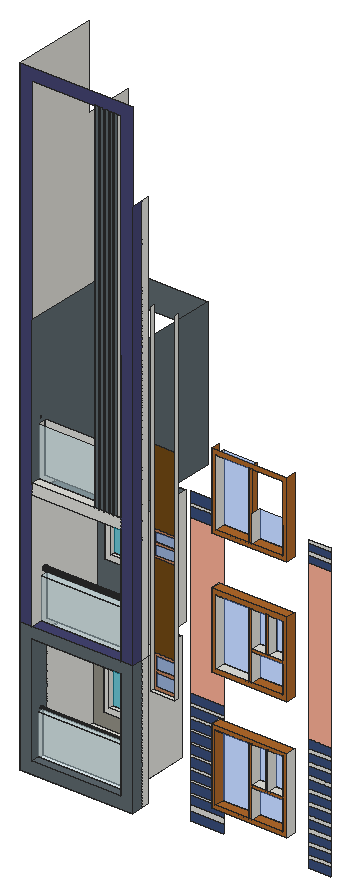
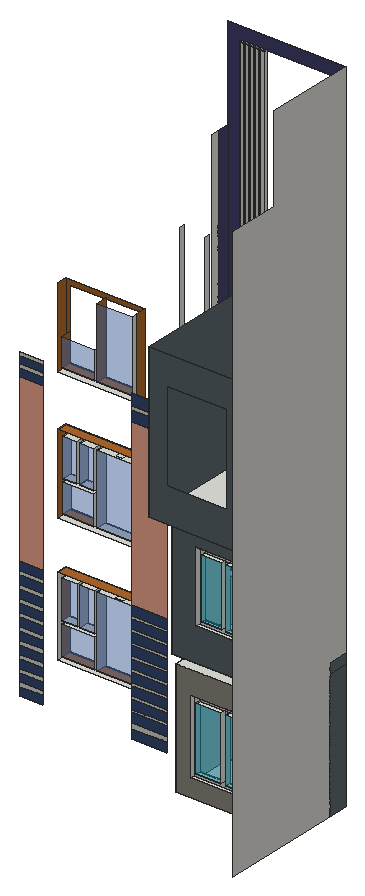
# SketchUp Ruby script. Lengths in inches.
U = 1.inch
M = Sketchup.active_model
def pt(a) = Geom::Point3d.new(a.map { |v| v * U })
def face(e, loops, mat)
  f = e.add_face(loops[0].map { |a| pt(a) })
  loops[1..].each { |l| e.add_face(l.map { |a| pt(a) }).erase! }
  f.material = f.back_material = mat if mat
  f
end
# faces: each face lists its corners as indices into pts; further lists are holes
def faces(e, pts, list, mat = nil) = list.each { |f| face(e, (f[0].is_a?(Array) ? f : [f]).map { |l| l.map { |i| pts[i] } }, mat) }
# xy, xz, yz: faces in a plane at the given z, y or x. An outline is a flat list of corners, or four numbers for a rectangle; further outlines are holes
def ring(l) = l.size == 4 ? [[l[0], l[1]], [l[2], l[1]], [l[2], l[3]], [l[0], l[3]]] : l.each_slice(2).to_a
def flat(e, list, mat, &to3) = list.each { |f| face(e, (f[0].is_a?(Array) ? f : [f]).map { |l| ring(l).map { |u, v| to3.(u, v) } }, mat) }
def xy(e, z, list, mat = nil) = flat(e, list, mat) { |x, y| [x, y, z] }
def xz(e, y, list, mat = nil) = flat(e, list, mat) { |x, z| [x, y, z] }
def yz(e, x, list, mat = nil) = flat(e, list, mat) { |y, z| [x, y, z] }
def lines(e, pts, list) = list.each { |a, b| e.add_line(pt(pts[a]), pt(pts[b])) }
# prism: a flat outline (further loops are holes) pulled along v
def prism(e, loops, v, mat = nil)
  f = face(e, loops, mat); d = Geom::Vector3d.new(v.map { |x| x * U })
  f.pushpull(f.normal.samedirection?(d) ? d.length : -d.length)
end
def box(e, o, s, mat = nil) = prism(e, [[o, [o[0] + s[0], o[1], o[2]], [o[0] + s[0], o[1] + s[1], o[2]], [o[0], o[1] + s[1], o[2]]]], [0, 0, s[2]], mat)
def at(x, y, z, deg = 0) = Geom::Transformation.translation(pt([x, y, z])) * Geom::Transformation.rotation(ORIGIN, Z_AXIS, deg.degrees)
def axes(o, x, y, z) = Geom::Transformation.new([*x, 0, *y, 0, *z, 0, *pt(o).to_a, 1])
def part(name) = M.definitions.add(name)
# library, detail: a bought-in or finely detailed component or shape, given as its bounding box
def library(name, o, s) = part(name).tap { |d| box(d.entities, o, s) }
def detail(e, o, s) = box(e.add_group.entities, o, s)
def put(e, d, t, mat = nil) = e.add_instance(d, t).tap { |i| i.material = mat if mat }
def group(e, t, mat = nil) = e.add_group.tap { |g| g.transformation = t; g.material = mat if mat }.entities
root = M.entities
M.materials.add("[Blinds Weave]").color = [114, 74, 20]
M.materials.add("[Color B02]").color = [255, 178, 153]
M.materials.add("[Color I02]").color = [68, 68, 114]
M.materials.add("[Formica Blue]").color = [58, 79, 124]
M.materials.add("[Formica Graystone]").color = [149, 146, 135]
M.materials.add("[Formica Speckled Grey]").color = [94, 105, 111]
M.materials.add("[Terrazzo Tile Light]").color = [219, 217, 210]
M.materials.add("[Translucent Glass Blue]").color = [100, 149, 237]
M.materials["[Translucent Glass Blue]"].alpha = 0.5
M.materials.add("[Translucent Glass Safety]").color = [204, 235, 244]
M.materials["[Translucent Glass Safety]"].alpha = 0.5
M.materials.add("[Translucent Glass Tinted]").color = [8, 201, 241]
M.materials["[Translucent Glass Tinted]"].alpha = 0.48
M.materials.add("[Wood Bamboo]").color = [177, 105, 43]
M.materials.add("[Wood Veneer 02]").color = [190, 128, 91]
xy(root,279.75,[[0,7.5,0,18.26,13.78,18.26,13.78,61.625,320.63,61.625,320.63,7.5]])
xy(root,313.07,[[33.32,45.54,287.32,227.125]])
xy(root,313.07,[[33.32,7.5,287.32,29.45]],"[Formica Speckled Grey]")
xy(root,360.6875,[[72.83,214.5625,246.76,227.125]])
xy(root,376.26,[[88.4,214.5625,150.48,227.125],[164.58,214.5625,231.1875,227.125]])
xy(root,378.36,[[552.31,0,767.87,28.0625]])
xy(root,389.26,[[563.2,0,660.09,28.0625],[667.35,0,756.97,28.0625]],"[Wood Bamboo]")
xy(root,429.69,[[33.32,29.45,287.32,45.54]],"[Translucent Glass Safety]")
xy(root,470.05,[[667.35,0,756.97,28.0625]])
xy(root,477.65,[[667.35,0,708.74,28.0625],[713.89,0,756.97,28.0625]])
xy(root,548.74,[[88.4,214.5625,150.48,227.125],[164.58,214.5625,231.1875,227.125]])
xy(root,564.3125,[[72.83,214.5625,246.76,227.125]])
xy(root,583.02,[[[563.2,0,660.09,28.0625],[593.19,6.08,612.69,23.46]],[667.35,0,708.74,28.0625],[713.89,0,756.97,28.0625],[593.19,6.08,612.69,23.46]])
xy(root,586.3125,[[345.55,40.625,414.87,53.5625]])
xy(root,593.92,[[552.31,0,767.87,28.0625]],"[Wood Bamboo]")
xy(root,626.26,[[0,7.5,33.32,61.625],[[33.32,7.5,287.32,61.625],[52.66,20.59,85.91,47.84],[228.16,20.59,261.41,47.84]],[52.66,20.59,85.91,47.84],[228.16,20.59,261.41,47.84],[33.32,61.625,287.32,227.125]])
xy(root,656.21,[[33.32,61.625,287.32,239.5625]])
xy(root,656.21,[[33.32,7.5,287.32,41.42]],"[Color I02]")
xy(root,726.11,[[552.31,0,767.87,28.0625]])
xy(root,738.9,[[565.1,0,660.09,28.0625]])
xy(root,738.9,[[669.04,0,755.07,28.0625]],"[Wood Bamboo]")
xy(root,745.45,[[66.75,227.8125,221.75,239.5625]])
xy(root,760.3,[[81.6,227.8125,139.43,239.5625],[152.36,227.8125,206.9,239.5625]])
xy(root,772.03,[[33.32,41.42,287.32,61.625]],"[Translucent Glass Safety]")
xy(root,817.79,[[669.04,0,755.07,28.0625]])
xy(root,825.96,[[669.04,0,707.54,28.0625],[715.14,0,755.07,28.0625]])
xy(root,925.04,[[81.6,227.8125,139.43,239.5625],[152.36,227.8125,206.9,239.5625]])
xy(root,928.88,[[[565.1,0,660.09,28.0625],[593.45,6.63,615.57,23.07]],[669.04,0,707.54,28.0625],[715.14,0,755.07,28.0625],[593.45,6.63,615.57,23.07]])
xy(root,939.89,[[66.75,227.8125,221.75,239.5625]])
xy(root,941.67,[[552.31,0,767.87,28.0625]],"[Wood Bamboo]")
xy(root,993.38,[[53.13,32.7,79.76,59.32],[228.95,32.7,255.57,59.32],[49.26,183.32,75.88,209.95],[228.95,183.32,255.57,209.95]])
xy(root,993.38,[[[33.32,7.5,287.32,239.5625],[53.13,32.7,79.76,59.32],[228.95,32.7,255.57,59.32],[228.95,183.32,255.57,209.95],[49.26,183.32,75.88,209.95]]],"[Formica Speckled Grey]")
xy(root,1023.34,[[33.32,7.5,213.36,7.5,213.36,17.375,224.6,17.375,224.6,7.5,227.11,7.5,227.11,17.375,238.35,17.375,238.35,7.5,241.05,7.5,241.05,17.375,252.29,17.375,252.29,7.5,255.11,7.5,255.11,17.375,266.35,17.375,266.35,7.5,269.11,7.5,269.11,17.375,280.35,17.375,280.35,7.5,287.32,7.5,287.32,31.52,33.32,31.52],[213.36,7.5,224.6,17.375],[227.11,7.5,238.35,17.375],[241.05,7.5,252.29,17.375],[255.11,7.5,266.35,17.375],
  [269.11,7.5,280.35,17.375],[33.32,55.75,287.32,318.5]])
xy(root,1082.8,[[552.31,0,767.87,28.0625]])
xy(root,1094.55,[[564.0625,0,660.09,28.0625],[667.45,0,756.11,28.0625]],"[Wood Bamboo]")
xz(root,0,[[[552.31,378.36,767.87,593.92],[563.2,389.26,756.97,583.02]],[660.09,389.26,667.35,583.02],[667.35,470.05,756.97,477.65],[708.74,477.65,713.89,583.02],[[552.31,726.11,767.87,941.67],[565.1,738.9,755.07,928.88]],
  [660.09,738.9,669.04,928.88],[669.04,817.79,755.07,825.96],[707.54,825.96,715.14,928.88],[[552.31,1082.8,767.87,1298.36],[564.0625,1094.55,756.11,1286.6]],[660.09,1094.55,667.45,1286.6]],"[Wood Bamboo]")
xz(root,7.5,[[33.32,993.38,287.32,1023.34]])
xz(root,7.5,[[0,656.21,33.32,656.21,33.32,2052.75,287.32,2052.75,287.32,656.21,320.63,656.21,320.63,2087.5625,0,2087.5625]],"[Color I02]")
xz(root,7.5,[[0,279.75,320.63,279.75,320.63,656.21,0,656.21,0,626.26,287.32,626.26,287.32,313.07,33.32,313.07,33.32,626.26,0,626.26],[213.36,1023.34,224.6,2052.75],[227.11,1023.34,238.35,2052.75],[241.05,1023.34,252.29,2052.75],[255.11,1023.34,266.35,2052.75],
  [269.11,1023.34,280.35,2052.75]],"[Formica Speckled Grey]")
xz(root,17.375,[[213.36,1023.34,224.6,2052.75],[227.11,1023.34,238.35,2052.75],[241.05,1023.34,252.29,2052.75],[255.11,1023.34,266.35,2052.75],[269.11,1023.34,280.35,2052.75]])
xz(root,28.0625,[[563.2,389.26,660.09,583.02],[667.35,389.26,756.97,470.05],[667.35,477.65,708.74,583.02],[713.89,477.65,756.97,583.02],[565.1,738.9,660.09,928.88],
  [669.04,738.9,755.07,817.79],[669.04,825.96,707.54,928.88],[715.14,825.96,755.07,928.88],[564.0625,1094.55,660.09,1286.6],[667.45,1094.55,756.11,1171.56]],"[Translucent Glass Blue]")
xz(root,29.45,[[33.32,313.07,287.32,429.69]],"[Translucent Glass Safety]")
xz(root,31.52,[[33.32,1023.34,287.32,1165.4]],"[Translucent Glass Safety]")
xz(root,41.42,[[33.32,656.21,287.32,772.03]],"[Translucent Glass Safety]")
xz(root,45.54,[[33.32,313.07,287.32,429.69]])
xz(root,53.5625,[[345.55,680.48,414.87,923.58],[345.55,998.27,414.87,1212.67]],"[Blinds Weave]")
xz(root,53.5625,[[353.15,593.91,407.27,630.07],[353.15,639.46,407.27,672.89],[352.13,930.16,408.29,958.03],[352.13,964.22,408.29,991.69]],"[Translucent Glass Blue]")
xz(root,53.5625,[[[345.55,586.3125,414.87,680.48],[353.15,593.91,407.27,672.89]],[353.15,630.07,407.27,639.46],[[345.55,923.58,414.87,998.27],[352.13,930.16,408.29,991.69]],[352.13,958.03,408.29,964.22]],"[Wood Veneer 02]")
xz(root,55.75,[[33.32,1023.34,287.32,1165.4]])
xz(root,61.625,[[782.27,302.4,843.32,312.28],[443.82,306.77,538.37,320.57],[782.27,335.77,843.32,346.28],[443.82,346.58,538.37,353.19],[782.27,369.77,843.32,380.28],
  [443.82,379.21,538.37,385.82],[782.27,403.77,843.32,414.28],[443.82,411.83,538.37,418.44],[782.27,437.77,843.32,448.28],[443.82,444.46,538.37,451.07],
  [782.27,471.77,843.32,482.28],[443.82,477.08,538.37,483.69],[782.27,505.77,843.32,516.28],[443.82,509.71,538.37,516.32],[782.27,539.77,843.32,550.28],
  [443.82,542.33,538.37,548.94],[782.27,573.77,843.32,584.28],[443.82,574.96,538.37,581.57],[33.32,656.21,287.32,772.03],[782.27,1079.01,843.32,1088.41],
  [443.82,1085.07,538.37,1094.19],[782.27,1109.47,843.32,1118.875]])
xz(root,61.625,[[443.82,607.58,538.37,1053.88],[782.27,607.77,843.32,1057.95]],"[Color B02]")
xz(root,61.625,[[782.27,278.91,843.32,302.4],[443.82,280.75,538.37,306.77],[782.27,312.28,843.32,335.77],[443.82,320.57,538.37,346.58],[782.27,346.28,843.32,369.77],
  [443.82,353.19,538.37,379.21],[782.27,380.28,843.32,403.77],[443.82,385.82,538.37,411.83],[782.27,414.28,843.32,437.77],[443.82,418.44,538.37,444.46],
  [782.27,448.28,843.32,471.77],[443.82,451.07,538.37,477.08],[782.27,482.28,843.32,505.77],[443.82,483.69,538.37,509.71],[782.27,516.28,843.32,539.77],
  [443.82,516.32,538.37,542.33],[443.82,548.94,538.37,574.96],[782.27,550.28,843.32,573.77],[443.82,581.57,538.37,607.58],[782.27,584.28,843.32,607.77],
  [443.82,1053.88,538.37,1085.07],[782.27,1057.95,843.32,1079.01],[782.27,1088.41,843.32,1109.47],[443.82,1094.19,538.37,1125.38]],"[Formica Blue]")
xz(root,214.5625,[[[72.83,360.6875,246.76,564.3125],[88.4,376.26,231.1875,548.74]],[150.48,376.26,164.58,548.74]])
xz(root,227.125,[[[33.32,313.07,287.32,626.26],[72.83,360.6875,246.76,564.3125]]],"[Formica Graystone]")
xz(root,227.125,[[88.4,376.26,150.48,548.74],[164.58,376.26,231.1875,548.74]],"[Translucent Glass Tinted]")
xz(root,227.8125,[[[66.75,745.45,221.75,939.89],[81.6,760.3,206.9,925.04]],[139.43,760.3,152.36,925.04]])
xz(root,239.5625,[[[33.32,656.21,287.32,993.38],[66.75,745.45,221.75,939.89]]],"[Formica Speckled Grey]")
xz(root,239.5625,[[81.6,760.3,139.43,925.04],[152.36,760.3,206.9,925.04]],"[Translucent Glass Tinted]")
xz(root,318.5,[[[33.32,1023.34,287.32,1439.76],[74.41,1117.04,237.41,1361.98]]],"[Formica Speckled Grey]")
yz(root,0,[[7.5,279.75,61.625,626.26],[7.5,626.26,61.625,656.21]],"[Formica Speckled Grey]")
yz(root,0,[[61.625,279.75,61.625,656.21,7.5,656.21,7.5,2087.5625,252.1,2087.5625,252.1,1852.125,391.54,1852.125,391.54,279.75]],"[Terrazzo Tile Light]")
yz(root,33.32,[[61.625,313.07,227.125,626.26],[[7.5,656.21,41.42,656.21,41.42,772.03,61.625,772.03,61.625,656.21,239.5625,656.21,239.5625,993.38,7.5,993.38],[50.17,783.1,48.47,783.32,46.89,783.98,45.53,785.02,44.49,786.38,43.83,787.97,43.61,789.66,43.83,791.36,44.49,792.94,45.53,794.3,46.89,795.35,48.47,796,50.17,796.23,51.87,796,53.45,795.35,54.8125,794.3,55.86,792.94,56.51,791.36,56.74,789.66,56.51,787.97,55.86,786.38,54.8125,785.02,53.45,783.98,51.87,783.32]]])
yz(root,33.32,[[[7.5,313.07,29.45,313.07,29.45,429.69,45.54,429.69,45.54,313.07,61.625,313.07,61.625,626.26,7.5,626.26],[37.49,435.16,36.68,435.27,35.93,435.58,35.28,436.08,34.78,436.72,34.47,437.48,34.37,438.28,34.47,439.09,34.78,439.85,35.28,440.49,35.93,440.99,36.68,441.3,37.49,441.41,38.3,441.3,39.05,440.99,39.7,440.49,40.2,439.85,40.51,439.09,40.62,438.28,40.51,437.48,40.2,436.72,39.7,436.08,39.05,435.58,38.3,435.27]],[[7.5,1023.34,31.52,1023.34,31.52,1165.4,55.75,1165.4,55.75,1023.34,318.5,1023.34,318.5,1439.76,7.5,1439.76],[40.12,1173.19,38.74,1173.37,37.46,1173.9,36.36,1174.75,35.52,1175.85,34.99,1177.13,34.81,1178.5,34.99,1179.88,35.52,1181.16,36.36,1182.26,37.46,1183.1,38.74,1183.63,40.12,1183.82,41.49,1183.63,42.77,1183.1,43.875,1182.26,44.72,1181.16,45.25,1179.88,45.43,1178.5,45.25,1177.13,44.72,1175.85,43.875,1174.75,42.77,1173.9,41.49,1173.37]]],"[Formica Speckled Grey]")
yz(root,66.75,[[227.8125,745.45,239.5625,939.89]])
yz(root,72.83,[[214.5625,360.6875,227.125,564.3125]])
yz(root,81.6,[[227.8125,760.3,239.5625,925.04]])
yz(root,88.4,[[214.5625,376.26,227.125,548.74]])
yz(root,139.43,[[227.8125,760.3,239.5625,925.04]])
yz(root,150.48,[[214.5625,376.26,227.125,548.74]])
yz(root,152.36,[[227.8125,760.3,239.5625,925.04]])
yz(root,164.58,[[214.5625,376.26,227.125,548.74]])
yz(root,206.9,[[227.8125,760.3,239.5625,925.04]])
yz(root,213.36,[[7.5,1023.34,17.375,2052.75]])
yz(root,221.75,[[227.8125,745.45,239.5625,939.89]])
yz(root,224.6,[[7.5,1023.34,17.375,2052.75]])
yz(root,227.11,[[7.5,1023.34,17.375,2052.75]])
yz(root,231.1875,[[214.5625,376.26,227.125,548.74]])
yz(root,238.35,[[7.5,1023.34,17.375,2052.75]])
yz(root,241.05,[[7.5,1023.34,17.375,2052.75]])
yz(root,246.76,[[214.5625,360.6875,227.125,564.3125]])
yz(root,252.29,[[7.5,1023.34,17.375,2052.75]])
yz(root,255.11,[[7.5,1023.34,17.375,2052.75]])
yz(root,266.35,[[7.5,1023.34,17.375,2052.75]])
yz(root,269.11,[[7.5,1023.34,17.375,2052.75]])
yz(root,280.35,[[7.5,1023.34,17.375,2052.75]])
yz(root,287.32,[[61.625,313.07,227.125,626.26],[37.49,435.16,38.3,435.27,39.05,435.58,39.7,436.08,40.2,436.72,40.51,437.48,40.62,438.28,40.51,439.09,40.2,439.85,39.7,440.49,39.05,440.99,38.3,441.3,37.49,441.41,36.68,441.3,35.93,440.99,35.28,440.49,34.78,439.85,34.47,439.09,34.37,438.28,34.47,437.48,34.78,436.72,35.28,436.08,35.93,435.58,36.68,435.27],[[7.5,656.21,7.5,993.38,239.5625,993.38,239.5625,656.21,61.625,656.21,61.625,772.03,41.42,772.03,41.42,656.21],[50.17,783.1,51.87,783.32,53.45,783.98,54.8125,785.02,55.86,786.38,56.51,787.97,56.74,789.66,56.51,791.36,55.86,792.94,54.8125,794.3,53.45,795.35,51.87,796,50.17,796.23,48.47,796,46.89,795.35,45.53,794.3,44.49,792.94,43.83,791.36,43.61,789.66,43.83,787.97,44.49,786.38,45.53,785.02,46.89,783.98,48.47,783.32]],[50.17,783.1,51.87,783.32,53.45,783.98,54.8125,785.02,55.86,786.38,56.51,787.97,56.74,789.66,56.51,791.36,55.86,792.94,54.8125,794.3,53.45,795.35,51.87,796,50.17,796.23,48.47,796,46.89,795.35,45.53,794.3,44.49,792.94,43.83,791.36,43.61,789.66,43.83,787.97,44.49,786.38,45.53,785.02,46.89,783.98,48.47,783.32]])
yz(root,287.32,[[[7.5,313.07,7.5,626.26,61.625,626.26,61.625,313.07,45.54,313.07,45.54,429.69,29.45,429.69,29.45,313.07],[37.49,435.16,38.3,435.27,39.05,435.58,39.7,436.08,40.2,436.72,40.51,437.48,40.62,438.28,40.51,439.09,40.2,439.85,39.7,440.49,39.05,440.99,38.3,441.3,37.49,441.41,36.68,441.3,35.93,440.99,35.28,440.49,34.78,439.85,34.47,439.09,34.37,438.28,34.47,437.48,34.78,436.72,35.28,436.08,35.93,435.58,36.68,435.27]],[[7.5,1023.34,7.5,1439.76,318.5,1439.76,318.5,1023.34,55.75,1023.34,55.75,1165.4,31.52,1165.4,31.52,1023.34],[40.12,1173.19,41.49,1173.37,42.77,1173.9,43.875,1174.75,44.72,1175.85,45.25,1177.13,45.43,1178.5,45.25,1179.88,44.72,1181.16,43.875,1182.26,42.77,1183.1,41.49,1183.63,40.12,1183.82,38.74,1183.63,37.46,1183.1,36.36,1182.26,35.52,1181.16,34.99,1179.88,34.81,1178.5,34.99,1177.13,35.52,1175.85,36.36,1174.75,37.46,1173.9,38.74,1173.37]]],"[Formica Speckled Grey]")
yz(root,320.63,[[40.625,279.75,61.625,656.21],[40.625,656.21,61.625,1831.875]])
yz(root,320.63,[[7.5,656.21,40.625,1831.875]],"[Color I02]")
yz(root,320.63,[[7.5,279.75,40.625,656.21]],"[Formica Speckled Grey]")
yz(root,345.55,[[40.625,586.3125,53.5625,1568.875]])
yz(root,414.87,[[40.625,586.3125,53.5625,1568.875]])
yz(root,552.31,[[0,378.36,28.0625,593.92],[0,726.11,28.0625,941.67]])
yz(root,552.31,[[0,1082.8,28.0625,1298.36]],"[Wood Bamboo]")
yz(root,563.2,[[0,389.26,28.0625,583.02]],"[Wood Bamboo]")
yz(root,564.0625,[[0,1094.55,28.0625,1286.6]])
yz(root,565.1,[[0,738.9,28.0625,928.88]])
yz(root,660.09,[[0,389.26,28.0625,583.02],[0,738.9,28.0625,928.88]])
yz(root,660.09,[[0,1094.55,28.0625,1286.6]],"[Wood Bamboo]")
yz(root,667.35,[[0,389.26,28.0625,470.05],[0,477.65,28.0625,583.02]])
yz(root,667.45,[[0,1094.55,28.0625,1171.56]])
yz(root,669.04,[[0,738.9,28.0625,817.79],[0,825.96,28.0625,928.88]])
yz(root,707.54,[[0,825.96,28.0625,828.46],[0,828.46,28.0625,928.88]])
yz(root,708.74,[[0,477.65,28.0625,583.02]])
yz(root,713.89,[[0,477.65,28.0625,583.02]])
yz(root,715.14,[[0,825.96,28.0625,928.88]])
yz(root,755.07,[[0,738.9,28.0625,817.79],[0,825.96,28.0625,928.88]])
yz(root,756.11,[[0,1094.55,28.0625,1171.56]],"[Wood Bamboo]")
yz(root,756.97,[[0,389.26,28.0625,470.05],[0,477.65,28.0625,583.02]],"[Wood Bamboo]")
yz(root,767.87,[[0,378.36,28.0625,593.92]])
yz(root,767.87,[[0,726.11,28.0625,941.67],[0,1082.8,28.0625,1298.36]],"[Wood Bamboo]")
p = [[287.32,37.49,435.16],[287.32,36.68,435.27],[33.32,36.68,435.27],[33.32,37.49,435.16],[287.32,38.3,435.27],[33.32,38.3,435.27],
  [287.32,35.93,435.58],[33.32,35.93,435.58],[287.32,39.05,435.58],[33.32,39.05,435.58],[287.32,35.28,436.08],[33.32,35.28,436.08],
  [287.32,39.7,436.08],[33.32,39.7,436.08],[287.32,34.78,436.72],[33.32,34.78,436.72],[287.32,40.2,436.72],[33.32,40.2,436.72],
  [287.32,34.47,437.48],[33.32,34.47,437.48],[287.32,40.51,437.48],[33.32,40.51,437.48],[287.32,34.37,438.28],[33.32,34.37,438.28],
  [287.32,40.62,438.28],[33.32,40.62,438.28],[287.32,34.47,439.09],[33.32,34.47,439.09],[287.32,40.51,439.09],[33.32,40.51,439.09],
  [287.32,34.78,439.85],[33.32,34.78,439.85],[287.32,40.2,439.85],[33.32,40.2,439.85],[287.32,35.28,440.49],[33.32,35.28,440.49],
  [287.32,39.7,440.49],[33.32,39.7,440.49],[287.32,35.93,440.99],[33.32,35.93,440.99],[287.32,39.05,440.99],[33.32,39.05,440.99],
  [287.32,36.68,441.3],[33.32,36.68,441.3],[287.32,38.3,441.3],[33.32,38.3,441.3],[287.32,37.49,441.41],[33.32,37.49,441.41],
  [287.32,50.17,783.1],[287.32,48.47,783.32],[33.32,48.47,783.32],[33.32,50.17,783.1],[287.32,51.87,783.32],[33.32,51.87,783.32],
  [287.32,46.89,783.98],[33.32,46.89,783.98],[287.32,53.45,783.98],[33.32,53.45,783.98],[287.32,45.53,785.02],[33.32,45.53,785.02],
  [287.32,54.8125,785.02],[33.32,54.8125,785.02],[287.32,44.49,786.38],[33.32,44.49,786.38],[287.32,55.86,786.38],[33.32,55.86,786.38],
  [287.32,43.83,787.97],[33.32,43.83,787.97],[287.32,56.51,787.97],[33.32,56.51,787.97],[287.32,43.61,789.66],[33.32,43.61,789.66],
  [287.32,56.74,789.66],[33.32,56.74,789.66],[287.32,43.83,791.36],[33.32,43.83,791.36],[287.32,56.51,791.36],[33.32,56.51,791.36],
  [287.32,44.49,792.94],[33.32,44.49,792.94],[287.32,55.86,792.94],[33.32,55.86,792.94],[287.32,45.53,794.3],[33.32,45.53,794.3],
  [287.32,54.8125,794.3],[33.32,54.8125,794.3],[287.32,46.89,795.35],[33.32,46.89,795.35],[287.32,53.45,795.35],[33.32,53.45,795.35],
  [287.32,48.47,796],[33.32,48.47,796],[287.32,51.87,796],[33.32,51.87,796],[287.32,50.17,796.23],[33.32,50.17,796.23]]
faces(root,p,[[0,1,2,3],[4,0,3,5],[1,6,7,2],[8,4,5,9],[6,10,11,7],[12,8,9,13],[10,14,15,11],[16,12,13,17],
  [14,18,19,15],[20,16,17,21],[18,22,23,19],[24,20,21,25],[22,26,27,23],[28,24,25,29],[26,30,31,27],[32,28,29,33],
  [30,34,35,31],[36,32,33,37],[34,38,39,35],[40,36,37,41],[38,42,43,39],[44,40,41,45],[42,46,47,43],[46,44,45,47],
  [48,49,50,51],[52,48,51,53],[49,54,55,50],[56,52,53,57],[54,58,59,55],[60,56,57,61],[58,62,63,59],[64,60,61,65],
  [62,66,67,63],[68,64,65,69],[66,70,71,67],[72,68,69,73],[70,74,75,71],[76,72,73,77],[74,78,79,75],[80,76,77,81],
  [78,82,83,79],[84,80,81,85],[82,86,87,83],[88,84,85,89],[86,90,91,87],[92,88,89,93],[90,94,95,91],[94,92,93,95]],"[Formica Graystone]")
